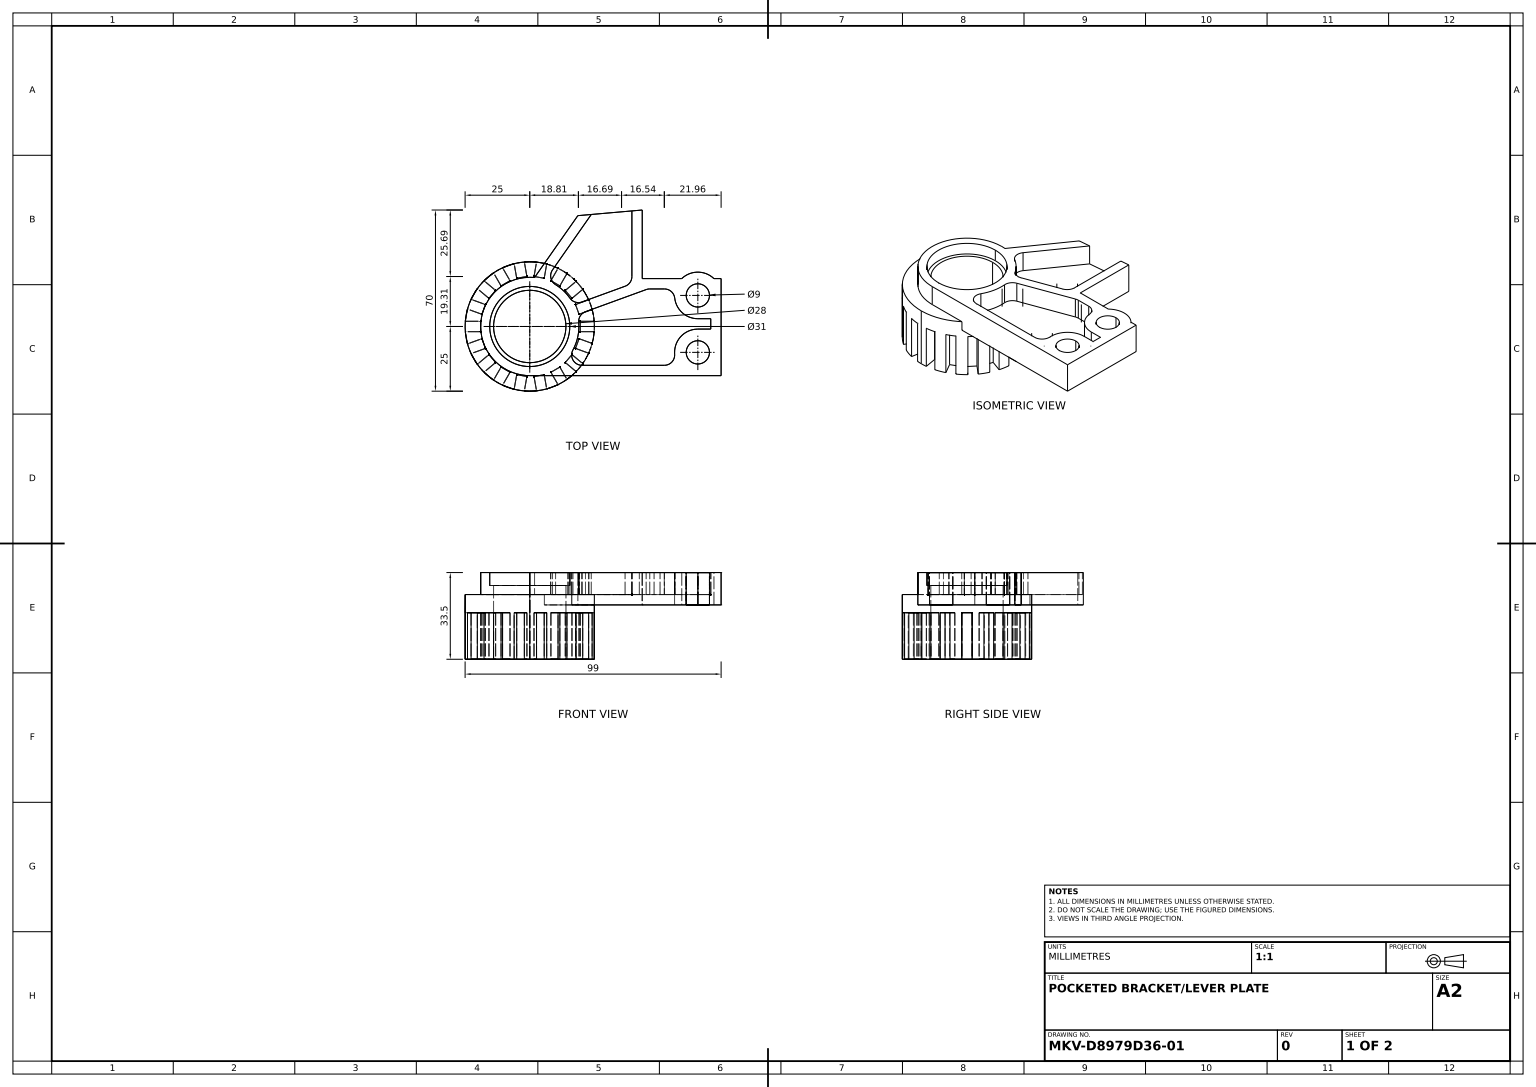
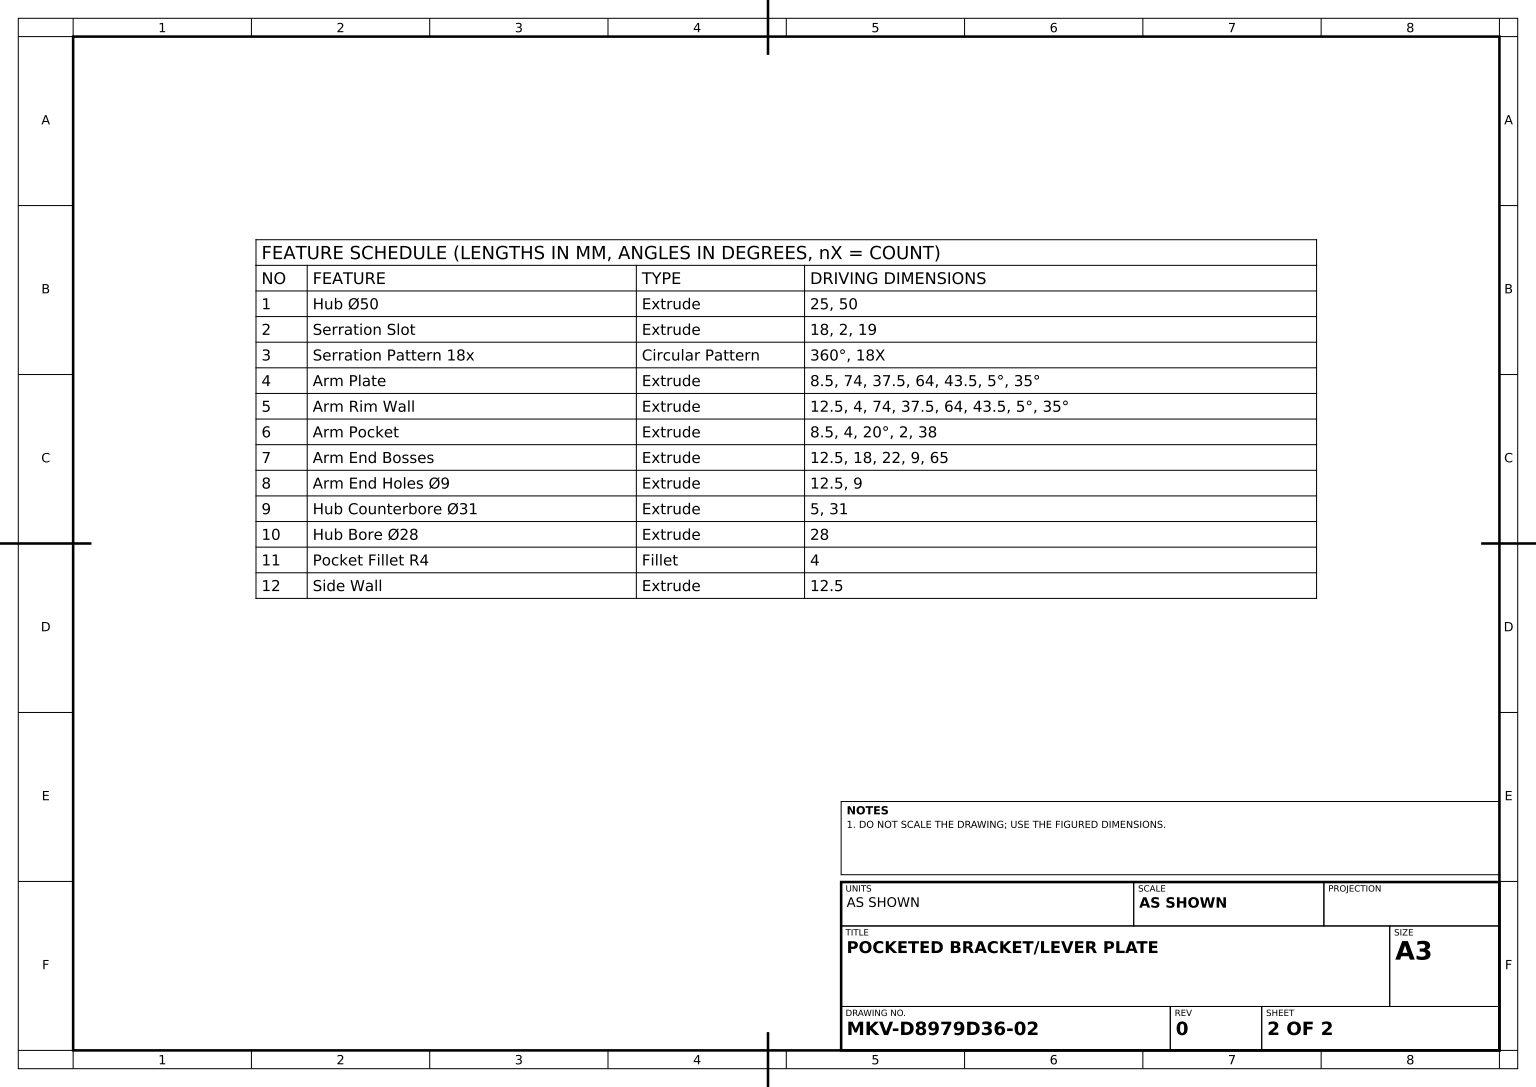
solid
v1 (0,8.5,-19)
v2 (0,0,-19)
e1 v1 v2 LINE
v3 (1.852058,8.5,-18.909518)
e2 v3 v1 CIRCLE(AX(P(0,8.5,0),D(0,1,0),D(0,0,1)),19)
v4 (1.852058,0,-18.909518)
e3 v3 v4 LINE
e4 v4 v2 CIRCLE(AX(P(0,0,0),D(0,1,0),D(0,0,1)),19)
face CYL(AX(P(0,8.5,0),D(0,-1,0),D(0,0,-1)),19) [-e1 -e2 e3 e4]
v5 (-7.632526,-25,17.689042)
v6 (-10.514782,-25,22.681256)
e5 v5 v6 LINE
v7 (-10.514782,-7,22.681256)
e6 v6 v7 LINE
v8 (-7.632526,-7,17.689042)
e7 v8 v7 LINE
e8 v8 v5 LINE
face PLANE(AX(P(-7.632526,-7,17.689042),D(0.866025404,0,0.5),D(0.5,0,-0.866025404))) rev [e5 e6 -e7 e8]
v9 (36.868081,0,-15.547239)
v10 (36.868081,8.5,-15.547239)
e9 v9 v10 LINE
v11 (39.5,8.5,-19.30601)
e10 v11 v10 CIRCLE(AX(P(35.5,8.5,-19.30601),D(0,-1,0),D(0,0,1)),4)
v12 (39.5,0,-19.30601)
e11 v12 v11 LINE
e12 v12 v9 CIRCLE(AX(P(35.5,0,-19.30601),D(0,-1,0),D(0,0,1)),4)
face CYL(AX(P(35.5,0,-19.30601),D(0,1,0),D(0,0,1)),4) rev [e9 -e10 -e11 e12]
v13 (65,-4,14.5)
v14 (65,8.5,14.5)
e13 v13 v14 LINE
v15 (65,8.5,5.5)
e14 v14 v15 CIRCLE(AX(P(65,8.5,10),D(0,1,0),D(0,0,1)),4.5)
v16 (65,-4,5.5)
e15 v16 v15 LINE
e16 v13 v16 CIRCLE(AX(P(65,-4,10),D(0,1,0),D(0,0,1)),4.5)
face CYL(AX(P(65,-4,10),D(0,1,0),D(0,0,1)),4.5) rev [e13 e14 -e15 -e16]
v17 (15.540712,8.5,-10.930977)
v18 (18.812441,8.5,-9.232235)
e17 v17 v18 CIRCLE(AX(P(18.812441,8.5,-13.232235),D(0,1,0),D(0,0,1)),4)
v19 (18.812441,0,-9.232235)
e18 v19 v18 LINE
v20 (15.540712,0,-10.930977)
e19 v20 v19 CIRCLE(AX(P(18.812441,0,-13.232235),D(0,1,0),D(0,0,1)),4)
e20 v20 v17 LINE
face CYL(AX(P(18.812441,0,-13.232235),D(0,1,0),D(0,0,1)),4) rev [e17 -e18 -e19 e20]
v21 (11.63832,-7,15.689042)
v22 (11.63832,-25,15.689042)
e21 v21 v22 LINE
v23 (14.385153,-25,20.446696)
e22 v22 v23 LINE
v24 (14.385153,-7,20.446696)
e23 v23 v24 LINE
e24 v21 v24 LINE
face PLANE(AX(P(11.63832,-7,15.689042),D(0.866025404,0,-0.5),D(-0.5,0,-0.866025404))) rev [e21 e22 e23 -e24]
v25 (0,-25,14)
v26 (0,-25,-14)
e25 v25 v26 CIRCLE(AX(P(0,-25,0),D(0,1,0),D(0,0,1)),14)
e26 v26 v25 CIRCLE(AX(P(0,-25,0),D(0,1,0),D(0,0,1)),14)
v27 (-13.205903,-25,13.91915)
v28 (-17.681074,-25,17.674264)
e27 v27 v28 LINE
v29 (-15.777054,-25,10.854972)
e28 v29 v27 LINE
v30 (-20.273632,-25,14.62805)
e29 v29 v30 LINE
v31 (-22.694147,-25,10.486929)
e30 v31 v30 CIRCLE(AX(P(0,-25,0),D(0,1,0),D(0,0,1)),25)
v32 (-17.153786,-25,8.470403)
e31 v32 v31 LINE
v33 (-18.521866,-25,4.711632)
e32 v33 v32 LINE
v34 (-24.0762,-25,6.733245)
e33 v33 v34 LINE
v35 (-24.919872,-25,2)
e34 v35 v34 CIRCLE(AX(P(0,-25,0),D(0,1,0),D(0,0,1)),25)
v36 (-19,-25,2)
e35 v36 v35 LINE
v37 (-19,-25,-2)
e36 v37 v36 LINE
v38 (-24.919872,-25,-2)
e37 v38 v37 LINE
v39 (-24.0762,-25,-6.733245)
e38 v39 v38 CIRCLE(AX(P(0,-25,0),D(0,1,0),D(0,0,1)),25)
v40 (-18.521866,-25,-4.711632)
e39 v40 v39 LINE
v41 (-17.153786,-25,-8.470403)
e40 v41 v40 LINE
v42 (-22.694147,-25,-10.486929)
e41 v41 v42 LINE
v43 (-20.273632,-25,-14.62805)
e42 v43 v42 CIRCLE(AX(P(0,-25,0),D(0,1,0),D(0,0,1)),25)
v44 (-15.777054,-25,-10.854972)
e43 v44 v43 LINE
v45 (-13.205903,-25,-13.91915)
e44 v45 v44 LINE
v46 (-17.681074,-25,-17.674264)
e45 v45 v46 LINE
v47 (-13.99771,-25,-20.713863)
e46 v47 v46 CIRCLE(AX(P(0,-25,0),D(0,1,0),D(0,0,1)),25)
v48 (-11.096628,-25,-15.689042)
e47 v48 v47 LINE
v49 (-7.632526,-25,-17.689042)
e48 v49 v48 LINE
v50 (-10.514782,-25,-22.681256)
e49 v49 v50 LINE
v51 (-6.037695,-25,-24.259972)
e50 v51 v50 CIRCLE(AX(P(0,-25,0),D(0,1,0),D(0,0,1)),25)
v52 (-5.045117,-25,-18.630782)
e51 v52 v51 LINE
v53 (-1.105886,-25,-19.325375)
e52 v53 v52 LINE
v54 (-2.091029,-25,-24.912398)
e53 v53 v54 LINE
v55 (0,-25,-25)
e54 v55 v54 CIRCLE(AX(P(0,-25,0),D(0,1,0),D(0,0,1)),25)
v56 (2.623822,-25,-24.86193)
e55 v56 v55 CIRCLE(AX(P(0,-25,0),D(0,1,0),D(0,0,1)),25)
v57 (1.647578,-25,-19.325375)
e56 v57 v56 LINE
v58 (5.586809,-25,-18.630782)
e57 v58 v57 LINE
v59 (6.555618,-25,-24.125171)
e58 v58 v59 LINE
v60 (10.939877,-25,-22.479304)
e59 v60 v59 CIRCLE(AX(P(0,-25,0),D(0,1,0),D(0,0,1)),25)
v61 (8.174218,-25,-17.689042)
e60 v61 v60 LINE
v62 (11.63832,-25,-15.689042)
e61 v62 v61 LINE
v63 (14.385153,-25,-20.446696)
e62 v62 v63 LINE
v64 (17.926296,-25,-17.425496)
e63 v64 v63 CIRCLE(AX(P(0,-25,0),D(0,1,0),D(0,0,1)),25)
v65 (13.747595,-25,-13.91915)
e64 v65 v64 LINE
v66 (16.318746,-25,-10.854972)
e65 v66 v65 LINE
v67 (20.476039,-25,-14.343355)
e66 v66 v67 LINE
v68 (22.771486,-25,-10.317919)
e67 v68 v67 CIRCLE(AX(P(0,-25,0),D(0,1,0),D(0,0,1)),25)
v69 (17.695477,-25,-8.470403)
e68 v69 v68 LINE
v70 (19.063558,-25,-4.711632)
e69 v70 v69 LINE
v71 (24.125594,-25,-6.554063)
e70 v70 v71 LINE
v72 (24.919872,-25,-2)
e71 v72 v71 CIRCLE(AX(P(0,-25,0),D(0,1,0),D(0,0,1)),25)
v73 (19.541692,-25,-2)
e72 v73 v72 LINE
v74 (19.541692,-25,2)
e73 v74 v73 LINE
v75 (24.919872,-25,2)
e74 v74 v75 LINE
v76 (24.125594,-25,6.554063)
e75 v76 v75 CIRCLE(AX(P(0,-25,0),D(0,1,0),D(0,0,1)),25)
v77 (19.063558,-25,4.711632)
e76 v77 v76 LINE
v78 (17.695477,-25,8.470403)
e77 v78 v77 LINE
v79 (22.771486,-25,10.317919)
e78 v78 v79 LINE
v80 (20.476039,-25,14.343355)
e79 v80 v79 CIRCLE(AX(P(0,-25,0),D(0,1,0),D(0,0,1)),25)
v81 (16.318746,-25,10.854972)
e80 v81 v80 LINE
v82 (13.747595,-25,13.91915)
e81 v82 v81 LINE
v83 (17.926296,-25,17.425496)
e82 v82 v83 LINE
e83 v23 v83 CIRCLE(AX(P(0,-25,0),D(0,1,0),D(0,0,1)),25)
v84 (8.174218,-25,17.689042)
e84 v84 v22 LINE
v85 (10.939877,-25,22.479304)
e85 v84 v85 LINE
v86 (6.555618,-25,24.125171)
e86 v86 v85 CIRCLE(AX(P(0,-25,0),D(0,1,0),D(0,0,1)),25)
v87 (5.586809,-25,18.630782)
e87 v87 v86 LINE
v88 (1.647578,-25,19.325375)
e88 v88 v87 LINE
v89 (2.623822,-25,24.86193)
e89 v88 v89 LINE
v90 (0,-25,25)
e90 v90 v89 CIRCLE(AX(P(0,-25,0),D(0,1,0),D(0,0,1)),25)
v91 (-2.091029,-25,24.912398)
e91 v91 v90 CIRCLE(AX(P(0,-25,0),D(0,1,0),D(0,0,1)),25)
v92 (-1.105886,-25,19.325375)
e92 v92 v91 LINE
v93 (-5.045117,-25,18.630782)
e93 v93 v92 LINE
v94 (-6.037695,-25,24.259972)
e94 v93 v94 LINE
e95 v6 v94 CIRCLE(AX(P(0,-25,0),D(0,1,0),D(0,0,1)),25)
v95 (-11.096628,-25,15.689042)
e96 v95 v5 LINE
v96 (-13.99771,-25,20.713863)
e97 v95 v96 LINE
e98 v28 v96 CIRCLE(AX(P(0,-25,0),D(0,1,0),D(0,0,1)),25)
face PLANE(AX(P(0,-25,0),D(0,1,0),D(0,0,1))) rev [e25 e26] [-e27 -e28 e29 -e30 -e31 -e32 e33 -e34 -e35 -e36 -e37 -e38 -e39 -e40 e41 -e42 -e43 -e44 e45 -e46 -e47 -e48 e49 -e50 -e51 -e52 e53 -e54 -e55 -e56 -e57 e58 -e59 -e60 -e61 e62 -e63 -e64 -e65 e66 -e67 -e68 -e69 e70 -e71 -e72 -e73 e74 -e75 -e76 -e77 e78 -e79 -e80 -e81 e82 -e83 -e22 -e84 e85 -e86 -e87 -e88 e89 -e90 -e91 -e92 -e93 e94 -e95 -e5 -e96 e97 -e98]
v97 (-15.777054,-7,10.854972)
e99 v97 v29 LINE
v98 (-20.273632,-7,14.62805)
e100 v98 v97 LINE
e101 v98 v30 LINE
face PLANE(AX(P(-15.777054,-7,10.854972),D(-0.64278761,0,-0.766044443),D(-0.766044443,0,0.64278761))) rev [-e29 -e99 -e100 e101]
e102 v16 v13 CIRCLE(AX(P(65,-4,10),D(0,1,0),D(0,0,1)),4.5)
e103 v15 v14 CIRCLE(AX(P(65,8.5,10),D(0,1,0),D(0,0,1)),4.5)
face CYL(AX(P(65,-4,10),D(0,1,0),D(0,0,1)),4.5) rev [-e102 e15 e103 -e13]
v99 (70,0,1)
v100 (65,0,1)
e104 v99 v100 LINE
v101 (65,8.5,1)
e105 v101 v100 LINE
v102 (70,8.5,1)
e106 v102 v101 LINE
e107 v99 v102 LINE
face PLANE(AX(P(65,-4,1),D(0,0,-1),D(-1,0,0))) [e104 -e105 -e106 -e107]
v103 (9.980466,8.5,-16.167569)
e108 v17 v103 CIRCLE(AX(P(0,8.5,0),D(0,1,0),D(0,0,1)),19)
v104 (9.980466,0,-16.167569)
e109 v20 v104 CIRCLE(AX(P(0,0,0),D(0,1,0),D(0,0,1)),19)
e110 v104 v103 LINE
face CYL(AX(P(0,0,0),D(0,1,0),D(0,0,1)),19) [-e108 -e20 e109 e110]
v105 (45.023259,8.5,-14.25877)
v106 (46.391339,8.5,-14.5)
e111 v105 v106 CIRCLE(AX(P(46.391339,8.5,-10.5),D(0,-1,0),D(0,0,1)),4)
v107 (45.023259,0,-14.25877)
e112 v107 v105 LINE
v108 (46.391339,0,-14.5)
e113 v107 v108 CIRCLE(AX(P(46.391339,0,-10.5),D(0,-1,0),D(0,0,1)),4)
e114 v108 v106 LINE
face CYL(AX(P(46.391339,0,-10.5),D(0,1,0),D(0,0,1)),4) rev [-e111 -e112 e113 e114]
v109 (21.548602,0,-5.714694)
v110 (18.931173,0,-1.615763)
e115 v109 v110 CIRCLE(AX(P(22.916683,0,-1.955924),D(0,1,0),D(0,0,1)),4)
v111 (16.686139,0,9.086957)
e116 v111 v110 CIRCLE(AX(P(0,0,0),D(0,1,0),D(0,0,1)),19)
v112 (20.19901,0,15)
e117 v111 v112 CIRCLE(AX(P(20.19901,0,11),D(0,1,0),D(0,0,1)),4)
v113 (52.038519,0,15)
e118 v112 v113 LINE
v114 (56.026667,0,10.692308)
e119 v113 v114 CIRCLE(AX(P(52.038519,0,11),D(0,1,0),D(0,0,1)),4)
e120 v100 v114 CIRCLE(AX(P(65,0,10),D(0,1,0),D(0,0,1)),9)
v115 (70,0,-3)
e121 v99 v115 LINE
v116 (65,0,-3)
e122 v116 v115 LINE
v117 (56.060112,0,-10.961538)
e123 v117 v116 CIRCLE(AX(P(65,0,-12),D(0,1,0),D(0,0,1)),9)
v118 (52.086828,0,-14.5)
e124 v117 v118 CIRCLE(AX(P(52.086828,0,-10.5),D(0,1,0),D(0,0,1)),4)
e125 v118 v108 LINE
e126 v109 v107 LINE
face PLANE(AX(P(0,0,0),D(0,1,0),D(0,0,1))) [e115 -e116 e117 e118 e119 -e120 -e104 e121 -e122 -e123 e124 e125 -e113 -e126]
v119 (65,-4,-7.5)
v120 (65,-4,-16.5)
e127 v119 v120 CIRCLE(AX(P(65,-4,-12),D(0,1,0),D(0,0,1)),4.5)
v121 (65,8.5,-7.5)
e128 v119 v121 LINE
v122 (65,8.5,-16.5)
e129 v121 v122 CIRCLE(AX(P(65,8.5,-12),D(0,1,0),D(0,0,1)),4.5)
e130 v120 v122 LINE
face CYL(AX(P(65,-4,-12),D(0,1,0),D(0,0,1)),4.5) rev [-e127 e128 e129 -e130]
v123 (43.5,8.5,-45)
v124 (43.5,-4,-45)
e131 v123 v124 LINE
v125 (18.595133,-4,-42.821106)
e132 v124 v125 LINE
v126 (18.595133,8.5,-42.821106)
e133 v126 v125 LINE
v127 (23.796892,8.5,-43.276201)
e134 v127 v126 LINE
v128 (23.796892,0,-43.276201)
e135 v128 v127 LINE
v129 (39.5,0,-44.650045)
e136 v129 v128 LINE
v130 (39.5,8.5,-44.650045)
e137 v129 v130 LINE
e138 v123 v130 LINE
face PLANE(AX(P(-3.576653,8.5,-40.881327),D(0.087155743,0,0.996194698),D(0.996194698,0,-0.087155743))) rev [e131 e132 -e133 -e134 -e135 -e136 e137 -e138]
v131 (20.180522,0,-9.473465)
e139 v131 v9 LINE
v132 (20.180522,8.5,-9.473465)
e140 v131 v132 LINE
e141 v132 v10 LINE
face PLANE(AX(P(-0.68404,0,-1.879385),D(0.342020143,0,0.939692621),D(0.939692621,0,-0.342020143))) rev [-e139 e140 e141 -e9]
v133 (17.926296,-7,17.425496)
v134 (13.747595,-7,13.91915)
e142 v133 v134 LINE
v135 (16.318746,-7,10.854972)
e143 v134 v135 LINE
v136 (20.476039,-7,14.343355)
e144 v135 v136 LINE
e145 v133 v136 CIRCLE(AX(P(0,-7,0),D(0,1,0),D(0,0,-1)),25)
face PLANE(AX(P(0.478326,-7,0.174096),D(0,-1,0),D(-0.64278761,0,0.766044443))) [e142 e143 e144 -e145]
v137 (24.125594,-7,-6.554063)
v138 (19.063558,-7,-4.711632)
e146 v137 v138 LINE
e147 v137 v71 LINE
e148 v138 v70 LINE
face PLANE(AX(P(19.063558,-7,-4.711632),D(0.342020143,0,0.939692621),D(0.939692621,0,-0.342020143))) rev [-e146 e147 -e70 -e148]
v139 (-5.045117,-7,18.630782)
v140 (-1.105886,-7,19.325375)
e149 v139 v140 LINE
v141 (-2.091029,-7,24.912398)
e150 v140 v141 LINE
v142 (-6.037695,-7,24.259972)
e151 v142 v141 CIRCLE(AX(P(0,-7,0),D(0,1,0),D(0,0,-1)),25)
e152 v142 v139 LINE
face PLANE(AX(P(0.223814,-7,0.266731),D(0,-1,0),D(-0.984807753,0,-0.173648178))) [e149 e150 -e151 e152]
v143 (-13.99771,-7,20.713863)
e153 v143 v7 CIRCLE(AX(P(0,-7,0),D(0,1,0),D(0,0,-1)),25)
e154 v142 v94 LINE
e155 v91 v141 LINE
v144 (0,0,25)
e156 v90 v144 LINE
v145 (0,0,-25)
e157 v145 v144 CIRCLE(AX(P(0,0,0),D(0,1,0),D(0,0,1)),25)
e158 v55 v145 LINE
v146 (-2.091029,-7,-24.912398)
e159 v146 v54 LINE
v147 (-6.037695,-7,-24.259972)
e160 v146 v147 CIRCLE(AX(P(0,-7,0),D(0,1,0),D(0,0,-1)),25)
e161 v51 v147 LINE
v148 (-10.514782,-7,-22.681256)
e162 v148 v50 LINE
v149 (-13.99771,-7,-20.713863)
e163 v148 v149 CIRCLE(AX(P(0,-7,0),D(0,1,0),D(0,0,-1)),25)
e164 v47 v149 LINE
v150 (-17.681074,-7,-17.674264)
e165 v150 v46 LINE
v151 (-20.273632,-7,-14.62805)
e166 v150 v151 CIRCLE(AX(P(0,-7,0),D(0,1,0),D(0,0,-1)),25)
e167 v43 v151 LINE
v152 (-22.694147,-7,-10.486929)
e168 v152 v42 LINE
v153 (-24.0762,-7,-6.733245)
e169 v152 v153 CIRCLE(AX(P(0,-7,0),D(0,1,0),D(0,0,-1)),25)
e170 v39 v153 LINE
v154 (-24.919872,-7,-2)
e171 v154 v38 LINE
v155 (-24.919872,-7,2)
e172 v155 v154 CIRCLE(AX(P(0,-7,0),D(0,-1,0),D(0,0,-1)),25)
e173 v155 v35 LINE
v156 (-24.0762,-7,6.733245)
e174 v156 v34 LINE
v157 (-22.694147,-7,10.486929)
e175 v156 v157 CIRCLE(AX(P(0,-7,0),D(0,1,0),D(0,0,-1)),25)
e176 v31 v157 LINE
v158 (-17.681074,-7,17.674264)
e177 v98 v158 CIRCLE(AX(P(0,-7,0),D(0,1,0),D(0,0,-1)),25)
e178 v28 v158 LINE
e179 v143 v96 LINE
face CYL(AX(P(0,-25,0),D(0,1,0),D(0,0,1)),25) [e153 -e6 e95 -e154 e151 -e155 e91 e156 -e157 -e158 e54 -e159 e160 -e161 e50 -e162 e163 -e164 e46 -e165 e166 -e167 e42 -e168 e169 -e170 e38 -e171 -e172 e173 e34 -e174 e175 -e176 e30 -e101 e177 -e178 e98 -e179]
e180 v140 v92 LINE
e181 v139 v93 LINE
face PLANE(AX(P(-1.105886,-7,19.325375),D(0.173648178,0,-0.984807753),D(-0.984807753,0,-0.173648178))) rev [-e180 -e149 e181 e93]
v159 (-11.096628,-7,15.689042)
e182 v159 v95 LINE
e183 v143 v159 LINE
face PLANE(AX(P(-11.096628,-7,15.689042),D(-0.866025404,0,-0.5),D(-0.5,0,0.866025404))) rev [-e182 -e183 e179 -e97]
v160 (13.747595,-7,-13.91915)
v161 (17.926296,-7,-17.425496)
e184 v160 v161 LINE
v162 (20.476039,-7,-14.343355)
e185 v162 v161 CIRCLE(AX(P(0,-7,0),D(0,1,0),D(0,0,-1)),25)
v163 (16.318746,-7,-10.854972)
e186 v162 v163 LINE
e187 v163 v160 LINE
face PLANE(AX(P(0.478326,-7,-0.174096),D(0,-1,0),D(0.64278761,0,0.766044443))) [e184 -e185 e186 e187]
v164 (56.026667,8.5,10.692308)
e188 v114 v164 LINE
e189 v101 v164 CIRCLE(AX(P(65,8.5,10),D(0,1,0),D(0,0,1)),9)
face CYL(AX(P(65,-4,10),D(0,1,0),D(0,0,1)),9) [e120 e188 -e189 e105]
v165 (8.174218,-7,17.689042)
e190 v165 v84 LINE
e191 v165 v21 LINE
face PLANE(AX(P(11.63832,-7,15.689042),D(-0.5,0,-0.866025404),D(-0.866025404,0,0.5))) rev [e190 e84 -e21 -e191]
v166 (24.919872,-7,2)
v167 (19.541692,-7,2)
e192 v166 v167 LINE
v168 (19.541692,-7,-2)
e193 v167 v168 LINE
v169 (24.919872,-7,-2)
e194 v168 v169 LINE
e195 v166 v169 CIRCLE(AX(P(0,-7,0),D(0,1,0),D(0,0,-1)),25)
face PLANE(AX(P(0.541692,-7,0),D(0,-1,0),D(0,0,1))) [e192 e193 e194 -e195]
v170 (11.63832,-7,-15.689042)
e196 v170 v62 LINE
v171 (14.385153,-7,-20.446696)
e197 v171 v170 LINE
e198 v171 v63 LINE
face PLANE(AX(P(11.63832,-7,-15.689042),D(0.866025404,0,0.5),D(0.5,0,-0.866025404))) rev [-e62 -e196 -e197 e198]
v172 (52.086828,8.5,-14.5)
e199 v118 v172 LINE
e200 v172 v106 LINE
face PLANE(AX(P(0,0,-14.5),D(0,0,-1),D(-1,0,0))) rev [e199 e200 -e114 -e125]
v173 (5.586809,-7,-18.630782)
v174 (1.647578,-7,-19.325375)
e201 v173 v174 LINE
v175 (2.623822,-7,-24.86193)
e202 v174 v175 LINE
v176 (6.555618,-7,-24.125171)
e203 v176 v175 CIRCLE(AX(P(0,-7,0),D(0,1,0),D(0,0,-1)),25)
e204 v176 v173 LINE
face PLANE(AX(P(0.317878,-7,-0.266731),D(0,-1,0),D(0.984807753,0,0.173648178))) [e201 e202 -e203 e204]
v177 (65,8.5,-3)
v178 (70,8.5,-3)
e205 v177 v178 LINE
e206 v177 v116 LINE
e207 v115 v178 LINE
face PLANE(AX(P(65,-4,-3),D(0,0,1),D(1,0,0))) [-e205 e206 e122 e207]
v179 (2.623822,-7,24.86193)
v180 (6.555618,-7,24.125171)
e208 v179 v180 CIRCLE(AX(P(0,-7,0),D(0,1,0),D(0,0,-1)),25)
v181 (1.647578,-7,19.325375)
e209 v179 v181 LINE
v182 (5.586809,-7,18.630782)
e210 v181 v182 LINE
e211 v182 v180 LINE
face PLANE(AX(P(0.317878,-7,0.266731),D(0,-1,0),D(-0.984807753,0,0.173648178))) [-e208 e209 e210 e211]
e212 v120 v119 CIRCLE(AX(P(65,-4,-12),D(0,1,0),D(0,0,1)),4.5)
v183 (43.5,-4,-18.5)
e213 v183 v124 LINE
v184 (58.77505,-4,-18.5)
e214 v184 v183 LINE
v185 (71.22495,-4,-18.5)
e215 v185 v184 CIRCLE(AX(P(65,-4,-12),D(0,1,0),D(0,0,1)),9)
v186 (74,-4,-18.5)
e216 v186 v185 LINE
v187 (74,-4,19)
e217 v187 v186 LINE
v188 (16.248077,-4,19)
e218 v188 v187 LINE
v189 (5.661829,-4,-24.350435)
e219 v189 v188 CIRCLE(AX(P(0,-4,0),D(0,-1,0),D(0,0,1)),25)
e220 v125 v189 LINE
face PLANE(AX(P(0,-4,0),D(0,1,0),D(0,0,1))) rev [e212 e127] [-e132 -e213 -e214 -e215 -e216 -e217 -e218 -e219 -e220] [e102 e16]
v190 (17.695477,-7,-8.470403)
v191 (22.771486,-7,-10.317919)
e221 v190 v191 LINE
e222 v190 v69 LINE
e223 v68 v191 LINE
face PLANE(AX(P(17.695477,-7,-8.470403),D(-0.342020143,0,-0.939692621),D(-0.939692621,0,0.342020143))) rev [-e221 e222 e68 e223]
e224 v138 v190 LINE
face PLANE(AX(P(17.695477,-7,-8.470403),D(-0.939692621,0,0.342020143),D(0.342020143,0,0.939692621))) rev [-e222 -e224 e148 e69]
e225 v56 v175 LINE
e226 v174 v57 LINE
face PLANE(AX(P(1.647578,-7,-19.325375),D(-0.984807753,0,-0.173648178),D(-0.173648178,0,0.984807753))) rev [e225 -e202 e226 e56]
v192 (-18.521866,-7,4.711632)
e227 v192 v33 LINE
e228 v156 v192 LINE
face PLANE(AX(P(-18.521866,-7,4.711632),D(-0.342020143,0,-0.939692621),D(-0.939692621,0,0.342020143))) rev [-e33 -e227 -e228 e174]
v193 (-11.096628,-7,-15.689042)
e229 v193 v149 LINE
e230 v193 v48 LINE
face PLANE(AX(P(-11.096628,-7,-15.689042),D(-0.866025404,0,0.5),D(0.5,0,0.866025404))) rev [-e229 e230 e47 e164]
e231 v12 v129 LINE
v194 (8.805009,0,-21.865574)
e232 v128 v194 LINE
e233 v194 v104 CIRCLE(AX(P(12.081617,0,-19.571268),D(0,1,0),D(0,0,1)),4)
e234 v19 v131 CIRCLE(AX(P(18.812441,0,-13.232235),D(0,1,0),D(0,0,1)),4)
face PLANE(AX(P(0,0,0),D(0,1,0),D(0,0,1))) [e139 -e12 e231 e136 e232 e233 -e109 e19 e234]
e235 v160 v65 LINE
e236 v64 v161 LINE
face PLANE(AX(P(13.747595,-7,-13.91915),D(-0.64278761,0,-0.766044443),D(-0.766044443,0,0.64278761))) rev [-e184 e235 e64 e236]
v195 (5.661829,0,-24.350435)
e237 v4 v195 LINE
e238 v195 v145 CIRCLE(AX(P(0,0,0),D(0,1,0),D(0,0,1)),25)
v196 (16.248077,0,19)
e239 v144 v196 CIRCLE(AX(P(0,0,0),D(0,1,0),D(0,0,1)),25)
v197 (0,0,19)
e240 v196 v197 LINE
e241 v2 v197 CIRCLE(AX(P(0,0,0),D(0,1,0),D(0,0,1)),19)
face PLANE(AX(P(0,0,0),D(0,1,0),D(0,0,1))) [-e4 e237 e238 e157 e239 e240 -e241]
v198 (8.174218,-7,-17.689042)
e242 v198 v61 LINE
e243 v170 v198 LINE
face PLANE(AX(P(8.174218,-7,-17.689042),D(-0.5,0,0.866025404),D(0.866025404,0,0.5))) rev [e61 -e242 -e243 e196]
v199 (8.805009,8.5,-21.865574)
e244 v194 v199 LINE
e245 v199 v103 CIRCLE(AX(P(12.081617,8.5,-19.571268),D(0,1,0),D(0,0,1)),4)
face CYL(AX(P(12.081617,0,-19.571268),D(0,1,0),D(0,0,1)),4) rev [e244 e245 -e110 -e233]
v200 (-17.153786,-7,8.470403)
e246 v200 v32 LINE
e247 v192 v200 LINE
face PLANE(AX(P(-17.153786,-7,8.470403),D(0.939692621,0,-0.342020143),D(-0.342020143,0,-0.939692621))) rev [e32 -e246 -e247 e227]
e248 v176 v59 LINE
e249 v173 v58 LINE
face PLANE(AX(P(5.586809,-7,-18.630782),D(0.984807753,0,0.173648178),D(0.173648178,0,-0.984807753))) rev [e248 -e58 -e249 -e204]
face PLANE(AX(P(-1.105886,-7,19.325375),D(0.984807753,0,0.173648178),D(0.173648178,0,-0.984807753))) rev [e155 -e150 e180 e92]
v201 (-13.205903,-7,13.91915)
e250 v201 v158 LINE
e251 v201 v27 LINE
face PLANE(AX(P(-13.205903,-7,13.91915),D(0.64278761,0,0.766044443),D(0.766044443,0,-0.64278761))) rev [e178 -e250 e251 e27]
e252 v181 v88 LINE
e253 v182 v87 LINE
face PLANE(AX(P(5.586809,-7,18.630782),D(-0.173648178,0,-0.984807753),D(-0.984807753,0,0.173648178))) rev [e252 e88 -e253 -e210]
face PLANE(AX(P(-5.045117,-7,18.630782),D(-0.984807753,0,-0.173648178),D(-0.173648178,0,0.984807753))) rev [-e94 -e181 -e152 e154]
v202 (-17.153786,-7,-8.470403)
v203 (-18.521866,-7,-4.711632)
e254 v202 v203 LINE
e255 v202 v41 LINE
e256 v203 v40 LINE
face PLANE(AX(P(-18.521866,-7,-4.711632),D(0.939692621,0,0.342020143),D(0.342020143,0,-0.939692621))) rev [-e254 e255 e40 -e256]
v204 (16.686139,8.5,9.086957)
e257 v111 v204 LINE
v205 (20.19901,8.5,15)
e258 v204 v205 CIRCLE(AX(P(20.19901,8.5,11),D(0,1,0),D(0,0,1)),4)
e259 v112 v205 LINE
face CYL(AX(P(20.19901,0,11),D(0,1,0),D(0,0,1)),4) rev [e257 e258 -e259 -e117]
e260 v72 v169 LINE
e261 v168 v73 LINE
face PLANE(AX(P(19.541692,-7,-2),D(0,0,-1),D(-1,0,0))) rev [e72 e260 -e194 e261]
v206 (17.695477,-7,8.470403)
e262 v206 v78 LINE
v207 (22.771486,-7,10.317919)
e263 v207 v206 LINE
e264 v207 v79 LINE
face PLANE(AX(P(17.695477,-7,8.470403),D(-0.342020143,0,0.939692621),D(0.939692621,0,0.342020143))) rev [-e78 -e262 -e263 e264]
face PLANE(AX(P(1.647578,-7,-19.325375),D(-0.173648178,0,0.984807753),D(0.984807753,0,0.173648178))) rev [-e226 -e201 e249 e57]
v208 (52.038519,8.5,15)
e265 v208 v113 LINE
e266 v164 v208 CIRCLE(AX(P(52.038519,8.5,11),D(0,-1,0),D(0,0,1)),4)
face CYL(AX(P(52.038519,-4,11),D(0,1,0),D(0,0,1)),4) rev [-e119 -e265 -e266 -e188]
e267 v97 v201 LINE
face PLANE(AX(P(0.063366,-7,0.174096),D(0,-1,0),D(-0.64278761,0,-0.766044443))) [e100 e267 e250 -e177]
e268 v163 v66 LINE
face PLANE(AX(P(13.747595,-7,-13.91915),D(-0.766044443,0,0.64278761),D(0.64278761,0,0.766044443))) rev [e268 e65 -e235 -e187]
v209 (-19,-7,-2)
v210 (-19,-7,2)
e269 v209 v210 LINE
e270 v210 v155 LINE
e271 v154 v209 LINE
face PLANE(AX(P(0,-7,0),D(0,-1,0),D(0,0,-1))) [e269 e270 e172 e271]
v211 (-5.045117,-7,-18.630782)
e272 v211 v147 LINE
v212 (-1.105886,-7,-19.325375)
e273 v146 v212 LINE
e274 v212 v211 LINE
face PLANE(AX(P(0.223814,-7,-0.266731),D(0,-1,0),D(0.984807753,0,-0.173648178))) [e272 -e160 e273 e274]
v213 (43.5,8.5,-18.5)
e275 v213 v183 LINE
v214 (58.77505,8.5,-18.5)
e276 v214 v213 LINE
e277 v214 v184 LINE
face PLANE(AX(P(0,8.5,-18.5),D(0,0,1),D(1,0,0))) rev [e214 -e275 -e276 e277]
v215 (10.939877,-7,-22.479304)
e278 v198 v215 LINE
e279 v60 v215 LINE
face PLANE(AX(P(8.174218,-7,-17.689042),D(-0.866025404,0,-0.5),D(-0.5,0,0.866025404))) rev [-e278 e242 e60 e279]
v216 (56.060112,8.5,-10.961538)
e280 v216 v177 CIRCLE(AX(P(65,8.5,-12),D(0,1,0),D(0,0,1)),9)
e281 v216 v117 LINE
face CYL(AX(P(65,-4,-12),D(0,1,0),D(0,0,1)),9) [-e206 -e280 e281 e123]
e282 v195 v189 LINE
e283 v126 v3 LINE
face PLANE(AX(P(-7.641818,8.5,-5.350858),D(0.819152044,0,0.573576436),D(0.573576436,0,-0.819152044))) rev [-e282 -e237 -e3 -e283 e133 e220]
e284 v86 v180 LINE
face PLANE(AX(P(5.586809,-7,18.630782),D(0.984807753,0,-0.173648178),D(-0.173648178,0,-0.984807753))) rev [e87 e284 -e211 e253]
v217 (0,3.5,15.5)
v218 (0,8.5,15.5)
e285 v217 v218 LINE
v219 (0,3.5,-15.5)
e286 v219 v217 CIRCLE(AX(P(0,3.5,0),D(0,1,0),D(0,0,1)),15.5)
v220 (0,8.5,-15.5)
e287 v219 v220 LINE
e288 v220 v218 CIRCLE(AX(P(0,8.5,0),D(0,1,0),D(0,0,1)),15.5)
face CYL(AX(P(0,3.5,0),D(0,1,0),D(0,0,1)),15.5) rev [-e285 -e286 e287 e288]
e289 v102 v178 LINE
face PLANE(AX(P(70,0,0),D(1,0,0),D(0,0,-1))) rev [e289 -e207 -e121 e107]
v221 (10.939877,-7,22.479304)
e290 v221 v165 LINE
e291 v221 v85 LINE
face PLANE(AX(P(8.174218,-7,17.689042),D(-0.866025404,0,0.5),D(0.5,0,0.866025404))) rev [-e290 e291 -e85 -e190]
v222 (74,8.5,-18.5)
e292 v222 v186 LINE
v223 (74,8.5,19)
e293 v223 v222 LINE
e294 v223 v187 LINE
face PLANE(AX(P(74,8.5,0),D(-1,0,0),D(0,0,1))) rev [e217 -e292 -e293 e294]
e295 v203 v153 LINE
face PLANE(AX(P(-18.521866,-7,-4.711632),D(-0.342020143,0,0.939692621),D(0.939692621,0,0.342020143))) rev [e256 e39 e170 -e295]
e296 v159 v8 LINE
face PLANE(AX(P(-7.632526,-7,17.689042),D(0.5,0,-0.866025404),D(-0.866025404,0,-0.5))) rev [e96 -e8 -e296 e182]
e297 v134 v82 LINE
e298 v135 v81 LINE
face PLANE(AX(P(16.318746,-7,10.854972),D(-0.766044443,0,-0.64278761),D(-0.64278761,0,0.766044443))) rev [-e143 e297 e81 -e298]
v224 (0,3.5,14)
v225 (0,3.5,-14)
e299 v224 v225 CIRCLE(AX(P(0,3.5,0),D(0,1,0),D(0,0,1)),14)
e300 v26 v225 LINE
e301 v25 v224 LINE
face CYL(AX(P(0,-25,0),D(0,1,0),D(0,0,1)),14) rev [e299 -e300 -e25 e301]
e302 v217 v219 CIRCLE(AX(P(0,3.5,0),D(0,1,0),D(0,0,1)),15.5)
e303 v218 v220 CIRCLE(AX(P(0,8.5,0),D(0,1,0),D(0,0,1)),15.5)
face CYL(AX(P(0,3.5,0),D(0,1,0),D(0,0,1)),15.5) rev [-e302 e285 e303 -e287]
e304 v200 v157 LINE
face PLANE(AX(P(0.016334,-7,0.092635),D(0,-1,0),D(-0.342020143,0,-0.939692621))) [-e175 e228 e247 e304]
face PLANE(AX(P(-17.153786,-7,8.470403),D(0.342020143,0,0.939692621),D(0.939692621,0,-0.342020143))) rev [e176 -e304 e246 e31]
e305 v225 v224 CIRCLE(AX(P(0,3.5,0),D(0,1,0),D(0,0,1)),14)
face PLANE(AX(P(0,3.5,0),D(0,1,0),D(0,0,1))) [-e299 -e305] [e286 e302]
v226 (0,8.5,19)
e306 v226 v197 LINE
e307 v1 v226 CIRCLE(AX(P(0,8.5,0),D(0,1,0),D(0,0,1)),19)
face CYL(AX(P(0,8.5,0),D(0,-1,0),D(0,0,-1)),19) [e1 e241 -e306 -e307]
face CYL(AX(P(0,-25,0),D(0,1,0),D(0,0,1)),14) rev [-e26 e300 e305 -e301]
e308 v179 v89 LINE
face PLANE(AX(P(1.647578,-7,19.325375),D(-0.984807753,0,0.173648178),D(0.173648178,0,0.984807753))) rev [-e209 e308 -e89 -e252]
e309 v122 v121 CIRCLE(AX(P(65,8.5,-12),D(0,1,0),D(0,0,1)),4.5)
face CYL(AX(P(65,-4,-12),D(0,1,0),D(0,0,1)),4.5) rev [e130 e309 -e128 -e212]
v227 (-13.205903,-7,-13.91915)
e310 v227 v45 LINE
e311 v150 v227 LINE
face PLANE(AX(P(-13.205903,-7,-13.91915),D(0.64278761,0,-0.766044443),D(-0.766044443,0,-0.64278761))) rev [-e310 -e311 e165 -e45]
v228 (24.125594,-7,6.554063)
e312 v207 v228 CIRCLE(AX(P(0,-7,0),D(0,1,0),D(0,0,-1)),25)
e313 v76 v228 LINE
e314 v166 v75 LINE
e315 v137 v191 CIRCLE(AX(P(0,-7,0),D(0,1,0),D(0,0,-1)),25)
e316 v162 v67 LINE
e317 v171 v215 CIRCLE(AX(P(0,-7,0),D(0,1,0),D(0,0,-1)),25)
e318 v188 v196 LINE
e319 v221 v24 CIRCLE(AX(P(0,-7,0),D(0,1,0),D(0,0,-1)),25)
e320 v133 v83 LINE
e321 v80 v136 LINE
face CYL(AX(P(0,-25,0),D(0,1,0),D(0,0,1)),25) [e79 -e264 e312 -e313 e75 -e314 e195 -e260 e71 -e147 e315 -e223 e67 -e316 e185 -e236 e63 -e198 e317 -e279 e59 -e248 e203 -e225 e55 e158 -e238 e282 e219 e318 -e239 -e156 e90 -e308 e208 -e284 e86 -e291 e319 -e23 e83 -e320 e145 -e321]
face PLANE(AX(P(16.318746,-7,10.854972),D(0.64278761,0,-0.766044443),D(-0.766044443,0,-0.64278761))) rev [-e144 e298 e80 e321]
v229 (71.22495,8.5,-18.5)
e322 v222 v229 LINE
e323 v185 v229 LINE
face PLANE(AX(P(0,8.5,-18.5),D(0,0,1),D(1,0,0))) rev [-e322 e292 e216 e323]
v230 (18.931173,8.5,-1.615763)
e324 v110 v230 LINE
e325 v204 v230 CIRCLE(AX(P(0,8.5,0),D(0,1,0),D(0,0,1)),19)
face CYL(AX(P(0,0,0),D(0,1,0),D(0,0,1)),19) [e116 e324 -e325 -e257]
face PLANE(AX(P(-13.205903,-7,13.91915),D(0.766044443,0,-0.64278761),D(-0.64278761,0,-0.766044443))) rev [-e251 -e267 e99 e28]
e326 v205 v208 LINE
v231 (21.548602,8.5,-5.714694)
e327 v231 v230 CIRCLE(AX(P(22.916683,8.5,-1.955924),D(0,1,0),D(0,0,1)),4)
e328 v231 v105 LINE
e329 v172 v216 CIRCLE(AX(P(52.086828,8.5,-10.5),D(0,-1,0),D(0,0,1)),4)
e330 v226 v223 LINE
e331 v229 v214 CIRCLE(AX(P(65,8.5,-12),D(0,1,0),D(0,0,1)),9)
e332 v213 v123 LINE
e333 v11 v130 LINE
e334 v18 v132 CIRCLE(AX(P(18.812441,8.5,-13.232235),D(0,1,0),D(0,0,1)),4)
e335 v127 v199 LINE
face PLANE(AX(P(0,8.5,0),D(0,1,0),D(0,0,1))) [-e303 -e288] [e266 -e326 -e258 e325 -e327 e328 e111 -e200 e329 e280 e205 -e289 e106 e189] [-e129 -e309] [-e103 -e14] [e283 e2 e307 e330 e293 e322 e331 e276 e332 e138 -e333 e10 -e141 -e334 -e17 e108 -e245 -e335 e134]
v232 (-15.777054,-7,-10.854972)
e336 v232 v151 LINE
e337 v232 v44 LINE
face PLANE(AX(P(-15.777054,-7,-10.854972),D(-0.64278761,0,0.766044443),D(0.766044443,0,0.64278761))) rev [e43 e167 -e336 e337]
face PLANE(AX(P(0.135423,-7,0.234559),D(0,-1,0),D(-0.866025404,0,-0.5))) [-e153 e183 e296 e7]
face CYL(AX(P(52.086828,-4,-10.5),D(0,1,0),D(0,0,1)),4) rev [-e199 -e124 -e281 -e329]
face PLANE(AX(P(43.5,8.5,0),D(-1,0,0),D(0,0,1))) rev [e275 e213 -e131 -e332]
face PLANE(AX(P(-4.365209,0,-3.056553),D(-0.819152044,0,-0.573576436),D(-0.573576436,0,0.819152044))) rev [-e244 -e232 e135 e335]
e338 v109 v231 LINE
face CYL(AX(P(22.916683,0,-1.955924),D(0,1,0),D(0,0,1)),4) rev [-e115 e338 e327 -e324]
face PLANE(AX(P(39.5,0,0),D(1,0,0),D(0,0,-1))) rev [-e231 e11 e333 -e137]
face PLANE(AX(P(0,8.5,19),D(0,0,-1),D(-1,0,0))) rev [-e240 -e318 e218 -e294 -e330 e306]
face PLANE(AX(P(16.318746,-7,-10.854972),D(0.64278761,0,0.766044443),D(0.766044443,0,-0.64278761))) rev [e316 -e66 -e268 -e186]
e339 v227 v232 LINE
face PLANE(AX(P(0.063366,-7,-0.174096),D(0,-1,0),D(0.64278761,0,-0.766044443))) [e336 -e166 e311 e339]
v233 (19.063558,-7,4.711632)
e340 v233 v228 LINE
e341 v233 v77 LINE
face PLANE(AX(P(19.063558,-7,4.711632),D(0.342020143,0,-0.939692621),D(-0.939692621,0,-0.342020143))) rev [e313 -e340 e341 e76]
e342 v212 v53 LINE
face PLANE(AX(P(-1.105886,-7,-19.325375),D(0.984807753,0,-0.173648178),D(-0.173648178,0,-0.984807753))) rev [-e53 -e342 -e273 e159]
e343 v209 v37 LINE
face PLANE(AX(P(-19,-7,-2),D(0,0,-1),D(-1,0,0))) rev [-e271 e171 e37 -e343]
e344 v152 v202 LINE
face PLANE(AX(P(0.016334,-7,-0.092635),D(0,-1,0),D(0.342020143,0,-0.939692621))) [e344 e254 e295 -e169]
face PLANE(AX(P(0,0,15),D(0,0,1),D(1,0,0))) rev [e326 e265 -e118 e259]
e345 v211 v52 LINE
face PLANE(AX(P(-5.045117,-7,-18.630782),D(-0.984807753,0,0.173648178),D(0.173648178,0,0.984807753))) rev [e161 -e272 e345 e51]
e346 v167 v74 LINE
face PLANE(AX(P(19.541692,-7,-2),D(-1,0,0),D(0,0,1))) rev [e346 e73 -e261 -e193]
face CYL(AX(P(18.812441,0,-13.232235),D(0,1,0),D(0,0,1)),4) rev [-e140 -e234 e18 e334]
e347 v210 v36 LINE
face PLANE(AX(P(-19,-7,2),D(0,0,1),D(1,0,0))) rev [e347 e35 -e173 -e270]
face PLANE(AX(P(13.747595,-7,13.91915),D(-0.64278761,0,0.766044443),D(0.766044443,0,0.64278761))) rev [e320 -e82 -e297 -e142]
face PLANE(AX(P(0.406269,-7,-0.234559),D(0,-1,0),D(0.866025404,0,0.5))) [e197 e243 e278 -e317]
v234 (-7.632526,-7,-17.689042)
e348 v148 v234 LINE
e349 v234 v193 LINE
face PLANE(AX(P(0.135423,-7,-0.234559),D(0,-1,0),D(0.866025404,0,-0.5))) [e348 e349 e229 -e163]
face PLANE(AX(P(-15.777054,-7,-10.854972),D(0.766044443,0,0.64278761),D(0.64278761,0,-0.766044443))) rev [e44 -e337 -e339 e310]
face PLANE(AX(P(-19,-7,2),D(1,0,0),D(0,0,-1))) rev [e36 -e347 -e269 e343]
face PLANE(AX(P(-17.153786,-7,-8.470403),D(0.342020143,0,-0.939692621),D(-0.939692621,0,-0.342020143))) rev [e168 -e41 -e255 -e344]
face PLANE(AX(P(19.541692,-7,2),D(0,0,1),D(1,0,0))) rev [e314 -e74 -e346 -e192]
e350 v206 v233 LINE
face PLANE(AX(P(19.063558,-7,4.711632),D(-0.939692621,0,-0.342020143),D(-0.342020143,0,0.939692621))) rev [e262 e77 -e341 -e350]
face PLANE(AX(P(0.525358,-7,-0.092635),D(0,-1,0),D(0.342020143,0,0.939692621))) [e146 e224 e221 -e315]
face PLANE(AX(P(0.68404,0,1.879385),D(0.342020143,0,0.939692621),D(0.939692621,0,-0.342020143))) [-e328 -e338 e126 e112]
face PLANE(AX(P(0.406269,-7,0.234559),D(0,-1,0),D(-0.866025404,0,0.5))) [e24 -e319 e290 e191]
face CYL(AX(P(65,-4,-12),D(0,1,0),D(0,0,1)),9) [-e331 -e323 e215 -e277]
e351 v234 v49 LINE
face PLANE(AX(P(-11.096628,-7,-15.689042),D(0.5,0,0.866025404),D(0.866025404,0,-0.5))) rev [-e349 e351 e48 -e230]
face PLANE(AX(P(0.525358,-7,0.092635),D(0,-1,0),D(-0.342020143,0,0.939692621))) [e263 e350 e340 -e312]
face PLANE(AX(P(-5.045117,-7,-18.630782),D(0.173648178,0,0.984807753),D(0.984807753,0,-0.173648178))) rev [e52 -e345 -e274 e342]
face PLANE(AX(P(-7.632526,-7,-17.689042),D(0.866025404,0,-0.5),D(-0.5,0,-0.866025404))) rev [-e348 e162 -e49 -e351]
